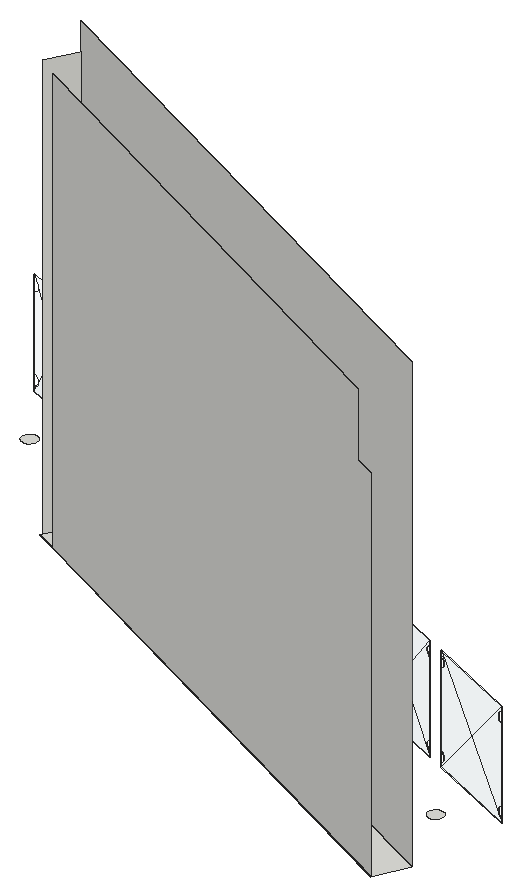
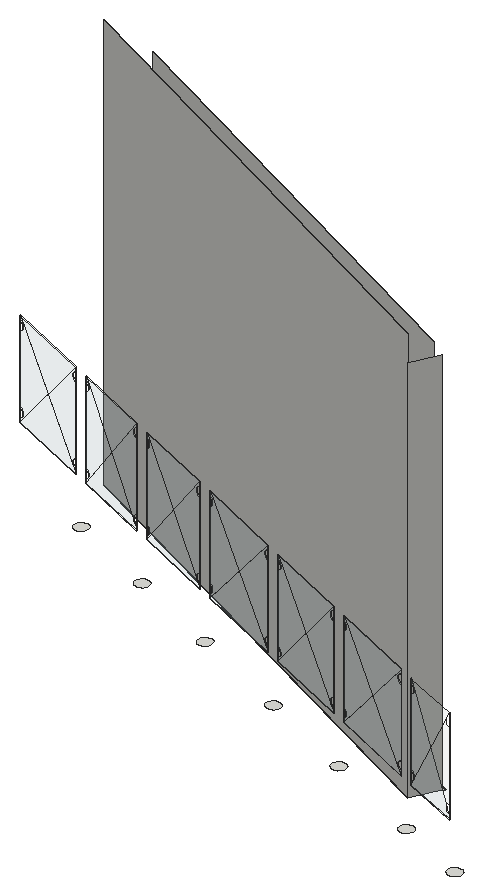
# SketchUp Ruby script. Lengths in inches.
U = 1.inch
M = Sketchup.active_model
def pt(a) = Geom::Point3d.new(a.map { |v| v * U })
def face(e, loops, mat)
  f = e.add_face(loops[0].map { |a| pt(a) })
  loops[1..].each { |l| e.add_face(l.map { |a| pt(a) }).erase! }
  f.material = f.back_material = mat if mat
  f
end
# faces: each face lists its corners as indices into pts; further lists are holes
def faces(e, pts, list, mat = nil) = list.each { |f| face(e, (f[0].is_a?(Array) ? f : [f]).map { |l| l.map { |i| pts[i] } }, mat) }
# xy, xz, yz: faces in a plane at the given z, y or x. An outline is a flat list of corners, or four numbers for a rectangle; further outlines are holes
def ring(l) = l.size == 4 ? [[l[0], l[1]], [l[2], l[1]], [l[2], l[3]], [l[0], l[3]]] : l.each_slice(2).to_a
def flat(e, list, mat, &to3) = list.each { |f| face(e, (f[0].is_a?(Array) ? f : [f]).map { |l| ring(l).map { |u, v| to3.(u, v) } }, mat) }
def xy(e, z, list, mat = nil) = flat(e, list, mat) { |x, y| [x, y, z] }
def xz(e, y, list, mat = nil) = flat(e, list, mat) { |x, z| [x, y, z] }
def yz(e, x, list, mat = nil) = flat(e, list, mat) { |y, z| [x, y, z] }
def lines(e, pts, list) = list.each { |a, b| e.add_line(pt(pts[a]), pt(pts[b])) }
# prism: a flat outline (further loops are holes) pulled along v
def prism(e, loops, v, mat = nil)
  f = face(e, loops, mat); d = Geom::Vector3d.new(v.map { |x| x * U })
  f.pushpull(f.normal.samedirection?(d) ? d.length : -d.length)
end
def box(e, o, s, mat = nil) = prism(e, [[o, [o[0] + s[0], o[1], o[2]], [o[0] + s[0], o[1] + s[1], o[2]], [o[0], o[1] + s[1], o[2]]]], [0, 0, s[2]], mat)
def at(x, y, z, deg = 0) = Geom::Transformation.translation(pt([x, y, z])) * Geom::Transformation.rotation(ORIGIN, Z_AXIS, deg.degrees)
def axes(o, x, y, z) = Geom::Transformation.new([*x, 0, *y, 0, *z, 0, *pt(o).to_a, 1])
def part(name) = M.definitions.add(name)
# library, detail: a bought-in or finely detailed component or shape, given as its bounding box
def library(name, o, s) = part(name).tap { |d| box(d.entities, o, s) }
def detail(e, o, s) = box(e.add_group.entities, o, s)
def put(e, d, t, mat = nil) = e.add_instance(d, t).tap { |i| i.material = mat if mat }
def group(e, t, mat = nil) = e.add_group.tap { |g| g.transformation = t; g.material = mat if mat }.entities
root = M.entities
M.materials.add("Glass_Safety_01").color = [204, 235, 244]
M.materials["Glass_Safety_01"].alpha = 0.1
M.materials.add("[Color_000]").color = [255, 255, 255]
xy(root,321.27,[[897.14,1046.9,900.47,1053.75,783.66,1110.47,780.62,1104.21,780.37,1103.68,784.86,1101.5,784.83,1101.43]])
xy(root,321.27,[[784.83,1101.43,784.86,1101.5,780.37,1103.68,780.33,1103.61]],"[Color_000]")
xy(root,321.86,[[893.19,1067.88,893.59,1067.97,893.96,1068.15,894.27,1068.42,894.5,1068.77,894.625,1069.16,894.65,1069.57,894.57,1069.97,894.38,1070.34,894.11,1070.64,893.77,1070.87,893.38,1071,892.97,1071.02,892.5625,1070.94,892.2,1070.76,891.89,1070.48,891.66,1070.14,891.53,1069.75,891.51,1069.34,891.59,1068.9375,891.78,1068.57,892.05,1068.26,892.39,1068.04,892.78,1067.91],[871.35,1077.4,871.75,1077.48,872.12,1077.66,872.43,1077.9375,872.65,1078.28,872.78,1078.67,872.81,1079.08,872.72,1079.48,872.54,1079.85,872.27,1080.16,871.92,1080.38,871.53,1080.51,871.12,1080.54,870.72,1080.46,870.35,1080.27,870.05,1080,869.82,1079.66,869.6875,1079.27,869.66,1078.85,869.75,1078.45,869.93,1078.08,870.2,1077.78,870.55,1077.55,870.9375,1077.42],[848.68,1087.27,849.08,1087.35,849.45,1087.54,849.76,1087.81,849.99,1088.15,850.12,1088.54,850.14,1088.95,850.06,1089.35,849.875,1089.72,849.6,1090.03,849.26,1090.26,848.87,1090.39,848.46,1090.41,848.05,1090.33,847.6875,1090.14,847.38,1089.87,847.15,1089.53,847.02,1089.14,847,1088.73,847.08,1088.32,847.27,1087.96,847.54,1087.65,847.88,1087.42,848.27,1087.29],[824.1,1097.98,824.5,1098.06,824.87,1098.24,825.18,1098.52,825.4,1098.86,825.53,1099.25,825.56,1099.66,825.47,1100.0625,825.29,1100.43,825.02,1100.74,824.67,1100.96,824.28,1101.09,823.87,1101.12,823.47,1101.03,823.1,1100.85,822.8,1100.58,822.57,1100.23,822.4375,1099.84,822.41,1099.43,822.5,1099.03,822.68,1098.66,822.95,1098.36,823.3,1098.13,823.6875,1098],[800.49,1108.26,800.89,1108.34,801.26,1108.53,801.57,1108.8,801.79,1109.14,801.92,1109.53,801.95,1109.94,801.86,1110.34,801.68,1110.71,801.41,1111.02,801.0625,1111.25,800.67,1111.375,800.26,1111.4,799.86,1111.32,799.49,1111.13,799.19,1110.86,798.96,1110.52,798.83,1110.125,798.8,1109.72,798.89,1109.3125,799.07,1108.95,799.34,1108.64,799.6875,1108.41,800.08,1108.28],
  [776.14,1118.86,776.55,1118.94,776.91,1119.13,777.22,1119.4,777.45,1119.74,777.58,1120.13,777.6,1120.54,777.52,1120.95,777.34,1121.31,777.0625,1121.62,776.72,1121.85,776.33,1121.98,775.92,1122,775.52,1121.92,775.15,1121.74,774.84,1121.46,774.61,1121.12,774.49,1120.73,774.46,1120.32,774.54,1119.92,774.73,1119.55,775,1119.24,775.34,1119.02,775.73,1118.89],[759.15,1125.91,759.3125,1125.94,759.56,1125.99,759.92,1126.18,760.23,1126.45,760.46,1126.79,760.59,1127.18,760.61,1127.59,760.53,1128,760.35,1128.36,760.07,1128.67,759.73,1128.9,759.34,1129.03,758.93,1129.05,758.53,1128.97,758.16,1128.79,757.85,1128.51,757.625,1128.17,757.49,1127.78,757.48,1127.57,757.47,1127.37,757.55,1126.97,757.74,1126.6,758.01,1126.29,758.35,1126.06,758.74,1125.93]])
xy(root,331.9,[[914.86,1059.86,894.71,1068.64,894.79,1068.82],[914.86,1059.86,894.79,1068.82,914.94,1060.04],[891.24,1070.15,872.85,1078.16,872.93,1078.34],[891.24,1070.15,872.93,1078.34,891.3125,1070.33],[869.39,1079.66,850.19,1088.03,850.27,1088.21],
  [869.39,1079.66,850.27,1088.21,869.47,1079.84],[846.73,1089.54,825.62,1098.73,825.7,1098.91],[846.73,1089.54,825.7,1098.91,846.8,1089.72],[822.14,1100.24,802,1109.01,802.08,1109.19],[822.14,1100.24,802.08,1109.19,822.22,1100.42],
  [798.53,1110.52,777.66,1119.61,777.74,1119.79],[798.53,1110.52,777.74,1119.79,798.61,1110.71],[774.18,1121.1,760.63,1126.72,760.7,1126.9],[774.18,1121.1,760.7,1126.9,774.25,1121.28]],"Glass_Safety_01")
p = [[784.83,1101.43,412.84],[784.83,1101.43,321.27],[897.14,1046.9,321.27],[897.14,1046.9,399.22],[892.64,1049.08,399.22],[892.64,1049.08,412.84],
  [783.66,1110.47,321.27],[783.66,1110.47,412.84],[783.66,1110.47,418.84],[900.47,1053.75,418.84],[900.47,1053.75,321.27],[780.62,1104.21,321.27],
  [780.62,1104.21,412.84],[914.86,1059.86,331.9],[914.86,1059.86,333],[914.61,1059.97,333.04],[914.375,1060.07,333.14],[914.17,1060.16,333.3125],
  [914.02,1060.23,333.53],[913.92,1060.27,333.79],[913.89,1060.28,334.0625],[913.92,1060.27,334.34],[914.02,1060.23,334.59],[914.17,1060.16,334.8125],
  [914.375,1060.07,334.98],[914.61,1059.97,335.09],[914.86,1059.86,335.125],[914.86,1059.86,351.28],[914.61,1059.97,351.32],[914.375,1060.07,351.43],
  [914.17,1060.16,351.59],[914.02,1060.23,351.8125],[913.92,1060.27,352.07],[913.89,1060.28,352.35],[913.92,1060.27,352.62],[914.02,1060.23,352.88],
  [914.17,1060.16,353.1],[914.375,1060.07,353.27],[914.61,1059.97,353.37],[914.86,1059.86,353.41],[914.86,1059.86,354.51],[894.71,1068.64,331.9],
  [894.71,1068.64,351.28],[894.71,1068.64,335.125],[894.84,1068.58,335.125],[895.1,1068.47,335.09],[895.33,1068.37,334.98],[895.53,1068.28,334.8125],
  [895.6875,1068.21,334.59],[895.79,1068.17,334.34],[895.82,1068.15,334.0625],[895.79,1068.17,333.79],[895.6875,1068.21,333.53],[895.53,1068.28,333.3125],
  [895.33,1068.37,333.14],[895.1,1068.47,333.04],[894.84,1068.58,333],[894.71,1068.64,333],[894.71,1068.64,354.51],[894.71,1068.64,353.41],
  [894.84,1068.58,353.41],[895.1,1068.47,353.37],[895.33,1068.37,353.27],[895.53,1068.28,353.1],[895.6875,1068.21,352.88],[895.79,1068.17,352.62],
  [895.82,1068.15,352.35],[895.79,1068.17,352.07],[895.6875,1068.21,351.8125],[895.53,1068.28,351.59],[895.33,1068.37,351.43],[895.1,1068.47,351.32],
  [894.84,1068.58,351.28],[914.94,1060.04,331.9],[914.94,1060.04,333],[914.94,1060.04,335.125],[914.94,1060.04,351.28],[914.94,1060.04,353.41],
  [914.94,1060.04,354.51],[914.69,1060.15,335.09],[914.46,1060.25,334.98],[914.25,1060.34,334.8125],[914.1,1060.41,334.59],[914,1060.45,334.34],
  [913.97,1060.46,334.0625],[914,1060.45,333.79],[914.1,1060.41,333.53],[914.25,1060.34,333.3125],[914.46,1060.25,333.14],[914.69,1060.15,333.04],
  [894.79,1068.82,354.51],[914.69,1060.15,353.37],[914.46,1060.25,353.27],[914.25,1060.34,353.1],[914.1,1060.41,352.88],[914,1060.45,352.62],
  [913.97,1060.46,352.35],[914,1060.45,352.07],[914.1,1060.41,351.8125],[914.25,1060.34,351.59],[914.46,1060.25,351.43],[914.69,1060.15,351.32],
  [894.79,1068.82,331.9],[894.79,1068.82,333],[894.92,1068.76,333],[895.18,1068.65,333.04],[895.41,1068.55,333.14],[895.61,1068.46,333.3125],
  [895.77,1068.39,333.53],[895.86,1068.35,333.79],[895.9,1068.33,334.0625],[895.86,1068.35,334.34],[895.77,1068.39,334.59],[895.61,1068.46,334.8125],
  [895.41,1068.55,334.98],[895.18,1068.65,335.09],[894.92,1068.76,335.125],[894.79,1068.82,335.125],[894.79,1068.82,351.28],[894.92,1068.76,351.28],
  [895.18,1068.65,351.32],[895.41,1068.55,351.43],[895.61,1068.46,351.59],[895.77,1068.39,351.8125],[895.86,1068.35,352.07],[895.9,1068.33,352.35],
  [895.86,1068.35,352.62],[895.77,1068.39,352.88],[895.61,1068.46,353.1],[895.41,1068.55,353.27],[895.18,1068.65,353.37],[894.92,1068.76,353.41],
  [894.79,1068.82,353.41],[891.24,1070.15,331.9],[891.24,1070.15,333],[890.98,1070.26,333.04],[890.75,1070.36,333.14],[890.55,1070.45,333.3125],
  [890.39,1070.52,333.53],[890.29,1070.56,333.79],[890.26,1070.57,334.0625],[890.29,1070.56,334.34],[890.39,1070.52,334.59],[890.55,1070.45,334.8125],
  [890.75,1070.36,334.98],[890.98,1070.26,335.09],[891.24,1070.15,335.125],[891.24,1070.15,351.28],[890.98,1070.26,351.32],[890.75,1070.36,351.43],
  [890.55,1070.45,351.59],[890.39,1070.52,351.8125],[890.29,1070.56,352.07],[890.26,1070.57,352.35],[890.29,1070.56,352.62],[890.39,1070.52,352.88],
  [890.55,1070.45,353.1],[890.75,1070.36,353.27],[890.98,1070.26,353.37],[891.24,1070.15,353.41],[891.24,1070.15,354.51],[872.85,1078.16,331.9],
  [872.85,1078.16,351.28],[872.85,1078.16,335.125],[873,1078.09,335.125],[873.25,1077.98,335.09],[873.49,1077.88,334.98],[873.69,1077.79,334.8125],
  [873.84,1077.72,334.59],[873.94,1077.68,334.34],[873.98,1077.67,334.0625],[873.94,1077.68,333.79],[873.84,1077.72,333.53],[873.69,1077.79,333.3125],
  [873.49,1077.88,333.14],[873.25,1077.98,333.04],[873,1078.09,333],[872.85,1078.16,333],[872.85,1078.16,354.51],[872.85,1078.16,353.41],
  [873,1078.09,353.41],[873.25,1077.98,353.37],[873.49,1077.88,353.27],[873.69,1077.79,353.1],[873.84,1077.72,352.88],[873.94,1077.68,352.62],
  [873.98,1077.67,352.35],[873.94,1077.68,352.07],[873.84,1077.72,351.8125],[873.69,1077.79,351.59],[873.49,1077.88,351.43],[873.25,1077.98,351.32],
  [873,1078.09,351.28],[891.3125,1070.33,331.9],[891.3125,1070.33,333],[891.3125,1070.33,335.125],[891.3125,1070.33,351.28],[891.3125,1070.33,353.41],
  [891.3125,1070.33,354.51],[891.0625,1070.44,335.09],[890.83,1070.54,334.98],[890.625,1070.63,334.8125],[890.47,1070.7,334.59],[890.37,1070.74,334.34],
  [890.34,1070.75,334.0625],[890.37,1070.74,333.79],[890.47,1070.7,333.53],[890.625,1070.63,333.3125],[890.83,1070.54,333.14],[891.0625,1070.44,333.04],
  [872.93,1078.34,354.51],[891.0625,1070.44,353.37],[890.83,1070.54,353.27],[890.625,1070.63,353.1],[890.47,1070.7,352.88],[890.37,1070.74,352.62],
  [890.34,1070.75,352.35],[890.37,1070.74,352.07],[890.47,1070.7,351.8125],[890.625,1070.63,351.59],[890.83,1070.54,351.43],[891.0625,1070.44,351.32],
  [872.93,1078.34,331.9],[872.93,1078.34,333],[873.08,1078.27,333],[873.33,1078.16,333.04],[873.57,1078.06,333.14],[873.77,1077.97,333.3125],
  [873.92,1077.9,333.53],[874.02,1077.86,333.79],[874.05,1077.85,334.0625],[874.02,1077.86,334.34],[873.92,1077.9,334.59],[873.77,1077.97,334.8125],
  [873.57,1078.06,334.98],[873.33,1078.16,335.09],[873.08,1078.27,335.125],[872.93,1078.34,335.125],[872.93,1078.34,351.28],[873.08,1078.27,351.28],
  [873.33,1078.16,351.32],[873.57,1078.06,351.43],[873.77,1077.97,351.59],[873.92,1077.9,351.8125],[874.02,1077.86,352.07],[874.05,1077.85,352.35],
  [874.02,1077.86,352.62],[873.92,1077.9,352.88],[873.77,1077.97,353.1],[873.57,1078.06,353.27],[873.33,1078.16,353.37],[873.08,1078.27,353.41],
  [872.93,1078.34,353.41],[869.39,1079.66,331.9],[869.39,1079.66,333],[869.14,1079.77,333.04],[868.9,1079.875,333.14],[868.7,1079.96,333.3125],
  [868.55,1080.03,333.53],[868.45,1080.07,333.79],[868.42,1080.09,334.0625],[868.45,1080.07,334.34],[868.55,1080.03,334.59],[868.7,1079.96,334.8125],
  [868.9,1079.875,334.98],[869.14,1079.77,335.09],[869.39,1079.66,335.125],[869.39,1079.66,351.28],[869.14,1079.77,351.32],[868.9,1079.875,351.43],
  [868.7,1079.96,351.59],[868.55,1080.03,351.8125],[868.45,1080.07,352.07],[868.42,1080.09,352.35],[868.45,1080.07,352.62],[868.55,1080.03,352.88],
  [868.7,1079.96,353.1],[868.9,1079.875,353.27],[869.14,1079.77,353.37],[869.39,1079.66,353.41],[869.39,1079.66,354.51],[850.19,1088.03,331.9],
  [850.19,1088.03,351.28],[850.19,1088.03,335.125],[850.33,1087.96,335.125],[850.59,1087.85,335.09],[850.82,1087.75,334.98],[851.02,1087.66,334.8125],
  [851.18,1087.6,334.59],[851.28,1087.55,334.34],[851.31,1087.54,334.0625],[851.28,1087.55,333.79],[851.18,1087.6,333.53],[851.02,1087.66,333.3125],
  [850.82,1087.75,333.14],[850.59,1087.85,333.04],[850.33,1087.96,333],[850.19,1088.03,333],[850.19,1088.03,354.51],[850.19,1088.03,353.41],
  [850.33,1087.96,353.41],[850.59,1087.85,353.37],[850.82,1087.75,353.27],[851.02,1087.66,353.1],[851.18,1087.6,352.88],[851.28,1087.55,352.62],
  [851.31,1087.54,352.35],[851.28,1087.55,352.07],[851.18,1087.6,351.8125],[851.02,1087.66,351.59],[850.82,1087.75,351.43],[850.59,1087.85,351.32],
  [850.33,1087.96,351.28],[869.47,1079.84,331.9],[869.47,1079.84,333],[869.47,1079.84,335.125],[869.47,1079.84,351.28],[869.47,1079.84,353.41],
  [869.47,1079.84,354.51],[869.22,1079.95,335.09],[868.98,1080.06,334.98],[868.78,1080.14,334.8125],[868.625,1080.21,334.59],[868.53,1080.25,334.34],
  [868.5,1080.27,334.0625],[868.53,1080.25,333.79],[868.625,1080.21,333.53],[868.78,1080.14,333.3125],[868.98,1080.06,333.14],[869.22,1079.95,333.04],
  [850.27,1088.21,354.51],[869.22,1079.95,353.37],[868.98,1080.06,353.27],[868.78,1080.14,353.1],[868.625,1080.21,352.88],[868.53,1080.25,352.62],
  [868.5,1080.27,352.35],[868.53,1080.25,352.07],[868.625,1080.21,351.8125],[868.78,1080.14,351.59],[868.98,1080.06,351.43],[869.22,1079.95,351.32],
  [850.27,1088.21,331.9],[850.27,1088.21,333],[850.41,1088.14,333],[850.67,1088.03,333.04],[850.9,1087.93,333.14],[851.1,1087.84,333.3125],
  [851.26,1087.78,333.53],[851.35,1087.73,333.79],[851.39,1087.72,334.0625],[851.35,1087.73,334.34],[851.26,1087.78,334.59],[851.1,1087.84,334.8125],
  [850.9,1087.93,334.98],[850.67,1088.03,335.09],[850.41,1088.14,335.125],[850.27,1088.21,335.125],[850.27,1088.21,351.28],[850.41,1088.14,351.28],
  [850.67,1088.03,351.32],[850.9,1087.93,351.43],[851.1,1087.84,351.59],[851.26,1087.78,351.8125],[851.35,1087.73,352.07],[851.39,1087.72,352.35],
  [851.35,1087.73,352.62],[851.26,1087.78,352.88],[851.1,1087.84,353.1],[850.9,1087.93,353.27],[850.67,1088.03,353.37],[850.41,1088.14,353.41],
  [850.27,1088.21,353.41],[846.73,1089.54,331.9],[846.73,1089.54,333],[846.47,1089.64,333.04],[846.24,1089.75,333.14],[846.04,1089.84,333.3125],
  [845.88,1089.9,333.53],[845.78,1089.95,333.79],[845.75,1089.96,334.0625],[845.78,1089.95,334.34],[845.88,1089.9,334.59],[846.04,1089.84,334.8125],
  [846.24,1089.75,334.98],[846.47,1089.64,335.09],[846.73,1089.54,335.125],[846.73,1089.54,351.28],[846.47,1089.64,351.32],[846.24,1089.75,351.43],
  [846.04,1089.84,351.59],[845.88,1089.9,351.8125],[845.78,1089.95,352.07],[845.75,1089.96,352.35],[845.78,1089.95,352.62],[845.88,1089.9,352.88],
  [846.04,1089.84,353.1],[846.24,1089.75,353.27],[846.47,1089.64,353.37],[846.73,1089.54,353.41],[846.73,1089.54,354.51],[825.62,1098.73,331.9],
  [825.62,1098.73,351.28],[825.62,1098.73,335.125],[825.75,1098.67,335.125],[826,1098.56,335.09],[826.24,1098.46,334.98],[826.44,1098.37,334.8125],
  [826.59,1098.3,334.59],[826.69,1098.26,334.34],[826.73,1098.25,334.0625],[826.69,1098.26,333.79],[826.59,1098.3,333.53],[826.44,1098.37,333.3125],
  [826.24,1098.46,333.14],[826,1098.56,333.04],[825.75,1098.67,333],[825.62,1098.73,333],[825.62,1098.73,354.51],[825.62,1098.73,353.41],
  [825.75,1098.67,353.41],[826,1098.56,353.37],[826.24,1098.46,353.27],[826.44,1098.37,353.1],[826.59,1098.3,352.88],[826.69,1098.26,352.62],
  [826.73,1098.25,352.35],[826.69,1098.26,352.07],[826.59,1098.3,351.8125],[826.44,1098.37,351.59],[826.24,1098.46,351.43],[826,1098.56,351.32],
  [825.75,1098.67,351.28],[846.8,1089.72,331.9],[846.8,1089.72,333],[846.8,1089.72,335.125],[846.8,1089.72,351.28],[846.8,1089.72,353.41],
  [846.8,1089.72,354.51],[846.55,1089.83,335.09],[846.32,1089.93,334.98],[846.11,1090.02,334.8125],[845.96,1090.08,334.59],[845.86,1090.125,334.34],
  [845.83,1090.14,334.0625],[845.86,1090.125,333.79],[845.96,1090.08,333.53],[846.11,1090.02,333.3125],[846.32,1089.93,333.14],[846.55,1089.83,333.04],
  [825.7,1098.91,354.51],[846.55,1089.83,353.37],[846.32,1089.93,353.27],[846.11,1090.02,353.1],[845.96,1090.08,352.88],[845.86,1090.125,352.62],
  [845.83,1090.14,352.35],[845.86,1090.125,352.07],[845.96,1090.08,351.8125],[846.11,1090.02,351.59],[846.32,1089.93,351.43],[846.55,1089.83,351.32],
  [825.7,1098.91,331.9],[825.7,1098.91,333],[825.83,1098.85,333],[826.08,1098.74,333.04],[826.32,1098.64,333.14],[826.52,1098.55,333.3125],
  [826.67,1098.48,333.53],[826.77,1098.44,333.79],[826.8,1098.43,334.0625],[826.77,1098.44,334.34],[826.67,1098.48,334.59],[826.52,1098.55,334.8125],
  [826.32,1098.64,334.98],[826.08,1098.74,335.09],[825.83,1098.85,335.125],[825.7,1098.91,335.125],[825.7,1098.91,351.28],[825.83,1098.85,351.28],
  [826.08,1098.74,351.32],[826.32,1098.64,351.43],[826.52,1098.55,351.59],[826.67,1098.48,351.8125],[826.77,1098.44,352.07],[826.8,1098.43,352.35],
  [826.77,1098.44,352.62],[826.67,1098.48,352.88],[826.52,1098.55,353.1],[826.32,1098.64,353.27],[826.08,1098.74,353.37],[825.83,1098.85,353.41],
  [825.7,1098.91,353.41],[822.14,1100.24,331.9],[822.14,1100.24,333],[821.89,1100.35,333.04],[821.65,1100.45,333.14],[821.45,1100.54,333.3125],
  [821.3,1100.61,333.53],[821.2,1100.65,333.79],[821.17,1100.67,334.0625],[821.2,1100.65,334.34],[821.3,1100.61,334.59],[821.45,1100.54,334.8125],
  [821.65,1100.45,334.98],[821.89,1100.35,335.09],[822.14,1100.24,335.125],[822.14,1100.24,351.28],[821.89,1100.35,351.32],[821.65,1100.45,351.43],
  [821.45,1100.54,351.59],[821.3,1100.61,351.8125],[821.2,1100.65,352.07],[821.17,1100.67,352.35],[821.2,1100.65,352.62],[821.3,1100.61,352.88],
  [821.45,1100.54,353.1],[821.65,1100.45,353.27],[821.89,1100.35,353.37],[822.14,1100.24,353.41],[822.14,1100.24,354.51],[802,1109.01,331.9],
  [802,1109.01,351.28],[802,1109.01,335.125],[802.14,1108.95,335.125],[802.39,1108.84,335.09],[802.63,1108.74,334.98],[802.83,1108.65,334.8125],
  [802.99,1108.59,334.59],[803.08,1108.54,334.34],[803.12,1108.53,334.0625],[803.08,1108.54,333.79],[802.99,1108.59,333.53],[802.83,1108.65,333.3125],
  [802.63,1108.74,333.14],[802.39,1108.84,333.04],[802.14,1108.95,333],[802,1109.01,333],[802,1109.01,354.51],[802,1109.01,353.41],
  [802.14,1108.95,353.41],[802.39,1108.84,353.37],[802.63,1108.74,353.27],[802.83,1108.65,353.1],[802.99,1108.59,352.88],[803.08,1108.54,352.62],
  [803.12,1108.53,352.35],[803.08,1108.54,352.07],[802.99,1108.59,351.8125],[802.83,1108.65,351.59],[802.63,1108.74,351.43],[802.39,1108.84,351.32],
  [802.14,1108.95,351.28],[822.22,1100.42,331.9],[822.22,1100.42,333],[822.22,1100.42,335.125],[822.22,1100.42,351.28],[822.22,1100.42,353.41],
  [822.22,1100.42,354.51],[821.97,1100.53,335.09],[821.73,1100.63,334.98],[821.53,1100.72,334.8125],[821.375,1100.79,334.59],[821.28,1100.83,334.34],
  [821.25,1100.85,334.0625],[821.28,1100.83,333.79],[821.375,1100.79,333.53],[821.53,1100.72,333.3125],[821.73,1100.63,333.14],[821.97,1100.53,333.04],
  [802.08,1109.19,354.51],[821.97,1100.53,353.37],[821.73,1100.63,353.27],[821.53,1100.72,353.1],[821.375,1100.79,352.88],[821.28,1100.83,352.62],
  [821.25,1100.85,352.35],[821.28,1100.83,352.07],[821.375,1100.79,351.8125],[821.53,1100.72,351.59],[821.73,1100.63,351.43],[821.97,1100.53,351.32],
  [802.08,1109.19,331.9],[802.08,1109.19,333],[802.22,1109.13,333],[802.47,1109.02,333.04],[802.71,1108.92,333.14],[802.91,1108.83,333.3125],
  [803.0625,1108.77,333.53],[803.16,1108.72,333.79],[803.19,1108.71,334.0625],[803.16,1108.72,334.34],[803.0625,1108.77,334.59],[802.91,1108.83,334.8125],
  [802.71,1108.92,334.98],[802.47,1109.02,335.09],[802.22,1109.13,335.125],[802.08,1109.19,335.125],[802.08,1109.19,351.28],[802.22,1109.13,351.28],
  [802.47,1109.02,351.32],[802.71,1108.92,351.43],[802.91,1108.83,351.59],[803.0625,1108.77,351.8125],[803.16,1108.72,352.07],[803.19,1108.71,352.35],
  [803.16,1108.72,352.62],[803.0625,1108.77,352.88],[802.91,1108.83,353.1],[802.71,1108.92,353.27],[802.47,1109.02,353.37],[802.22,1109.13,353.41],
  [802.08,1109.19,353.41],[798.53,1110.52,331.9],[798.53,1110.52,333],[798.28,1110.63,333.04],[798.04,1110.74,333.14],[797.84,1110.83,333.3125],
  [797.6875,1110.89,333.53],[797.59,1110.93,333.79],[797.56,1110.95,334.0625],[797.59,1110.93,334.34],[797.6875,1110.89,334.59],[797.84,1110.83,334.8125],
  [798.04,1110.74,334.98],[798.28,1110.63,335.09],[798.53,1110.52,335.125],[798.53,1110.52,351.28],[798.28,1110.63,351.32],[798.04,1110.74,351.43],
  [797.84,1110.83,351.59],[797.6875,1110.89,351.8125],[797.59,1110.93,352.07],[797.56,1110.95,352.35],[797.59,1110.93,352.62],[797.6875,1110.89,352.88],
  [797.84,1110.83,353.1],[798.04,1110.74,353.27],[798.28,1110.63,353.37],[798.53,1110.52,353.41],[798.53,1110.52,354.51],[777.66,1119.61,331.9],
  [777.66,1119.61,351.28],[777.66,1119.61,335.125],[777.8,1119.56,335.125],[778.05,1119.45,335.09],[778.28,1119.34,334.98],[778.49,1119.26,334.8125],
  [778.64,1119.1875,334.59],[778.74,1119.15,334.34],[778.77,1119.13,334.0625],[778.74,1119.15,333.79],[778.64,1119.1875,333.53],[778.49,1119.26,333.3125],
  [778.28,1119.34,333.14],[778.05,1119.45,333.04],[777.8,1119.56,333],[777.66,1119.61,333],[777.66,1119.61,354.51],[777.66,1119.61,353.41],
  [777.8,1119.56,353.41],[778.05,1119.45,353.37],[778.28,1119.34,353.27],[778.49,1119.26,353.1],[778.64,1119.1875,352.88],[778.74,1119.15,352.62],
  [778.77,1119.13,352.35],[778.74,1119.15,352.07],[778.64,1119.1875,351.8125],[778.49,1119.26,351.59],[778.28,1119.34,351.43],[778.05,1119.45,351.32],
  [777.8,1119.56,351.28],[798.61,1110.71,331.9],[798.61,1110.71,333],[798.61,1110.71,335.125],[798.61,1110.71,351.28],[798.61,1110.71,353.41],
  [798.61,1110.71,354.51],[798.36,1110.82,335.09],[798.12,1110.92,334.98],[797.92,1111.01,334.8125],[797.77,1111.07,334.59],[797.67,1111.12,334.34],
  [797.64,1111.13,334.0625],[797.67,1111.12,333.79],[797.77,1111.07,333.53],[797.92,1111.01,333.3125],[798.12,1110.92,333.14],[798.36,1110.82,333.04],
  [777.74,1119.79,354.51],[798.36,1110.82,353.37],[798.12,1110.92,353.27],[797.92,1111.01,353.1],[797.77,1111.07,352.88],[797.67,1111.12,352.62],
  [797.64,1111.13,352.35],[797.67,1111.12,352.07],[797.77,1111.07,351.8125],[797.92,1111.01,351.59],[798.12,1110.92,351.43],[798.36,1110.82,351.32],
  [777.74,1119.79,331.9],[777.74,1119.79,333],[777.875,1119.74,333],[778.13,1119.625,333.04],[778.36,1119.52,333.14],[778.56,1119.4375,333.3125],
  [778.72,1119.37,333.53],[778.82,1119.33,333.79],[778.85,1119.3125,334.0625],[778.82,1119.33,334.34],[778.72,1119.37,334.59],[778.56,1119.4375,334.8125],
  [778.36,1119.52,334.98],[778.13,1119.625,335.09],[777.875,1119.74,335.125],[777.74,1119.79,335.125],[777.74,1119.79,351.28],[777.875,1119.74,351.28],
  [778.13,1119.625,351.32],[778.36,1119.52,351.43],[778.56,1119.4375,351.59],[778.72,1119.37,351.8125],[778.82,1119.33,352.07],[778.85,1119.3125,352.35],
  [778.82,1119.33,352.62],[778.72,1119.37,352.88],[778.56,1119.4375,353.1],[778.36,1119.52,353.27],[778.13,1119.625,353.37],[777.875,1119.74,353.41],
  [777.74,1119.79,353.41],[774.18,1121.1,335.125],[774.18,1121.1,351.28],[773.92,1121.2,351.32],[773.68,1121.3,351.43],[773.48,1121.38,351.59],
  [773.33,1121.45,351.8125],[773.23,1121.49,352.07],[773.19,1121.5,352.35],[773.23,1121.49,352.62],[773.33,1121.45,352.88],[773.48,1121.38,353.1],
  [773.68,1121.3,353.27],[773.92,1121.2,353.37],[774.18,1121.1,353.41],[774.18,1121.1,354.51],[761.77,1126.24,333.81],[761.77,1126.24,333.79],
  [761.67,1126.28,333.53],[761.52,1126.35,333.3125],[761.43,1126.38,333.24],[760.63,1126.72,331.9],[774.18,1121.1,331.9],[774.18,1121.1,333],
  [773.92,1121.2,333.04],[773.68,1121.3,333.14],[773.48,1121.38,333.3125],[773.33,1121.45,333.53],[773.23,1121.49,333.79],[773.19,1121.5,334.0625],
  [773.23,1121.49,334.34],[773.33,1121.45,334.59],[773.48,1121.38,334.8125],[773.68,1121.3,334.98],[773.92,1121.2,335.09],[774.25,1121.28,331.9],
  [774.25,1121.28,333],[774.25,1121.28,335.125],[774.25,1121.28,351.28],[774.25,1121.28,353.41],[774.25,1121.28,354.51],[774,1121.38,335.09],
  [773.76,1121.48,334.98],[773.56,1121.57,334.8125],[773.4,1121.63,334.59],[773.3,1121.67,334.34],[773.27,1121.68,334.0625],[773.3,1121.67,333.79],
  [773.4,1121.63,333.53],[773.56,1121.57,333.3125],[773.76,1121.48,333.14],[774,1121.38,333.04],[761.85,1126.42,352.6],[761.85,1126.42,352.62],
  [761.75,1126.47,352.88],[761.59,1126.53,353.1],[761.51,1126.5625,353.17],[760.7,1126.9,354.51],[774,1121.38,353.37],[773.76,1121.48,353.27],
  [773.56,1121.57,353.1],[773.4,1121.63,352.88],[773.3,1121.67,352.62],[773.27,1121.68,352.35],[773.3,1121.67,352.07],[773.4,1121.63,351.8125],
  [773.56,1121.57,351.59],[773.76,1121.48,351.43],[774,1121.38,351.32],[760.7,1126.9,335.125],[760.7,1126.9,351.28],[760.9,1126.82,351.28],
  [761.15,1126.71,351.32],[761.39,1126.61,351.43],[761.59,1126.53,351.59],[761.75,1126.47,351.8125],[761.85,1126.42,352.07],[761.88,1126.41,352.35],
  [760.7,1126.9,331.9],[760.7,1126.9,333],[760.9,1126.82,333],[761.15,1126.71,333.04],[761.39,1126.61,333.14],[761.59,1126.53,333.3125],
  [761.75,1126.47,333.53],[761.85,1126.42,333.79],[761.88,1126.41,334.0625],[761.85,1126.42,334.34],[761.75,1126.47,334.59],[761.59,1126.53,334.8125],
  [761.39,1126.61,334.98],[761.15,1126.71,335.09],[760.9,1126.82,335.125],[761.3125,1126.43,333.14],[761.08,1126.53,333.04],[760.82,1126.64,333],
  [760.63,1126.72,333],[760.63,1126.72,335.125],[760.63,1126.72,351.28],[760.63,1126.72,353.41],[760.63,1126.72,354.51],[760.7,1126.9,353.41]]
faces(root,p,[[0,1,2,3,4,5],[6,7,8,9,10],[6,11,12,7]])
faces(root,p,[[13,14,15,16,17,18,19,20,21,22,23,24,25,26,27,28,29,30,31,32,33,34,35,36,37,38,39,40,41],[42,43,44,45,46,47,48,49,50,51,52,53,54,55,56,57,41,40,58,59,60,61,62,63,64,65,66,67,68,69,70,71,72],[13,73,74,75,76,77,78,40,39,27,26,14],[76,75,79,80,81,82,83,84,85,86,87,88,89,74,73,90,78,77,91,92,93,94,95,96,97,98,99,100,101],[102,103,104,105,106,107,108,109,110,111,112,113,114,115,116,117,118,119,120,121,122,123,124,125,126,127,128,129,130,131,132,90,73],[102,41,57,43,42,59,58,90,132,118,117,103],[133,134,135,136,137,138,139,140,141,142,143,144,145,146,147,148,149,150,151,152,153,154,155,156,157,158,159,160,161],[162,163,164,165,166,167,168,169,170,171,172,173,174,175,176,177,161,160,178,179,180,181,182,183,184,185,186,187,188,189,190,191,192],
  [133,193,194,195,196,197,198,160,159,147,146,134],[196,195,199,200,201,202,203,204,205,206,207,208,209,194,193,210,198,197,211,212,213,214,215,216,217,218,219,220,221],[222,223,224,225,226,227,228,229,230,231,232,233,234,235,236,237,238,239,240,241,242,243,244,245,246,247,248,249,250,251,252,210,193],[222,161,177,163,162,179,178,210,252,238,237,223],[253,254,255,256,257,258,259,260,261,262,263,264,265,266,267,268,269,270,271,272,273,274,275,276,277,278,279,280,281],[282,283,284,285,286,287,288,289,290,291,292,293,294,295,296,297,281,280,298,299,300,301,302,303,304,305,306,307,308,309,310,311,312],[253,313,314,315,316,317,318,280,279,267,266,254],[316,315,319,320,321,322,323,324,325,326,327,328,329,314,313,330,318,317,331,332,333,334,335,336,337,338,339,340,341],
  [342,343,344,345,346,347,348,349,350,351,352,353,354,355,356,357,358,359,360,361,362,363,364,365,366,367,368,369,370,371,372,330,313],[342,281,297,283,282,299,298,330,372,358,357,343],[373,374,375,376,377,378,379,380,381,382,383,384,385,386,387,388,389,390,391,392,393,394,395,396,397,398,399,400,401],[402,403,404,405,406,407,408,409,410,411,412,413,414,415,416,417,401,400,418,419,420,421,422,423,424,425,426,427,428,429,430,431,432],[373,433,434,435,436,437,438,400,399,387,386,374],[436,435,439,440,441,442,443,444,445,446,447,448,449,434,433,450,438,437,451,452,453,454,455,456,457,458,459,460,461],[462,463,464,465,466,467,468,469,470,471,472,473,474,475,476,477,478,479,480,481,482,483,484,485,486,487,488,489,490,491,492,450,433],[462,401,417,403,402,419,418,450,492,478,477,463],
  [493,494,495,496,497,498,499,500,501,502,503,504,505,506,507,508,509,510,511,512,513,514,515,516,517,518,519,520,521],[522,523,524,525,526,527,528,529,530,531,532,533,534,535,536,537,521,520,538,539,540,541,542,543,544,545,546,547,548,549,550,551,552],[493,553,554,555,556,557,558,520,519,507,506,494],[556,555,559,560,561,562,563,564,565,566,567,568,569,554,553,570,558,557,571,572,573,574,575,576,577,578,579,580,581],[582,583,584,585,586,587,588,589,590,591,592,593,594,595,596,597,598,599,600,601,602,603,604,605,606,607,608,609,610,611,612,570,553],[582,521,537,523,522,539,538,570,612,598,597,583],[613,614,615,616,617,618,619,620,621,622,623,624,625,626,627,628,629,630,631,632,633,634,635,636,637,638,639,640,641],[642,643,644,645,646,647,648,649,650,651,652,653,654,655,656,657,641,640,658,659,660,661,662,663,664,665,666,667,668,669,670,671,672],
  [613,673,674,675,676,677,678,640,639,627,626,614],[676,675,679,680,681,682,683,684,685,686,687,688,689,674,673,690,678,677,691,692,693,694,695,696,697,698,699,700,701],[702,703,704,705,706,707,708,709,710,711,712,713,714,715,716,717,718,719,720,721,722,723,724,725,726,727,728,729,730,731,732,690,673],[702,641,657,643,642,659,658,690,732,718,717,703],[733,734,735,736,737,738,739,740,741,742,743,744,745,746,747,748,749,750,751,752,753,754,755,756,757,758,759,760,761,762,763,764,765,766],[754,767,768,769,770,771,772,747,746,734,733,755],[770,769,773,774,775,776,777,778,779,780,781,782,783,768,767,784,785,786,787,788,789,772,771,790,791,792,793,794,795,796,797,798,799,800],[801,802,803,804,805,806,807,808,809,784,767,810,811,812,813,814,815,816,817,818,819,820,821,822,823,824],
  [753,752,825,826,827,828],[810,753,828,829,830,831,832,789,833,802,801,811]],"Glass_Safety_01")
